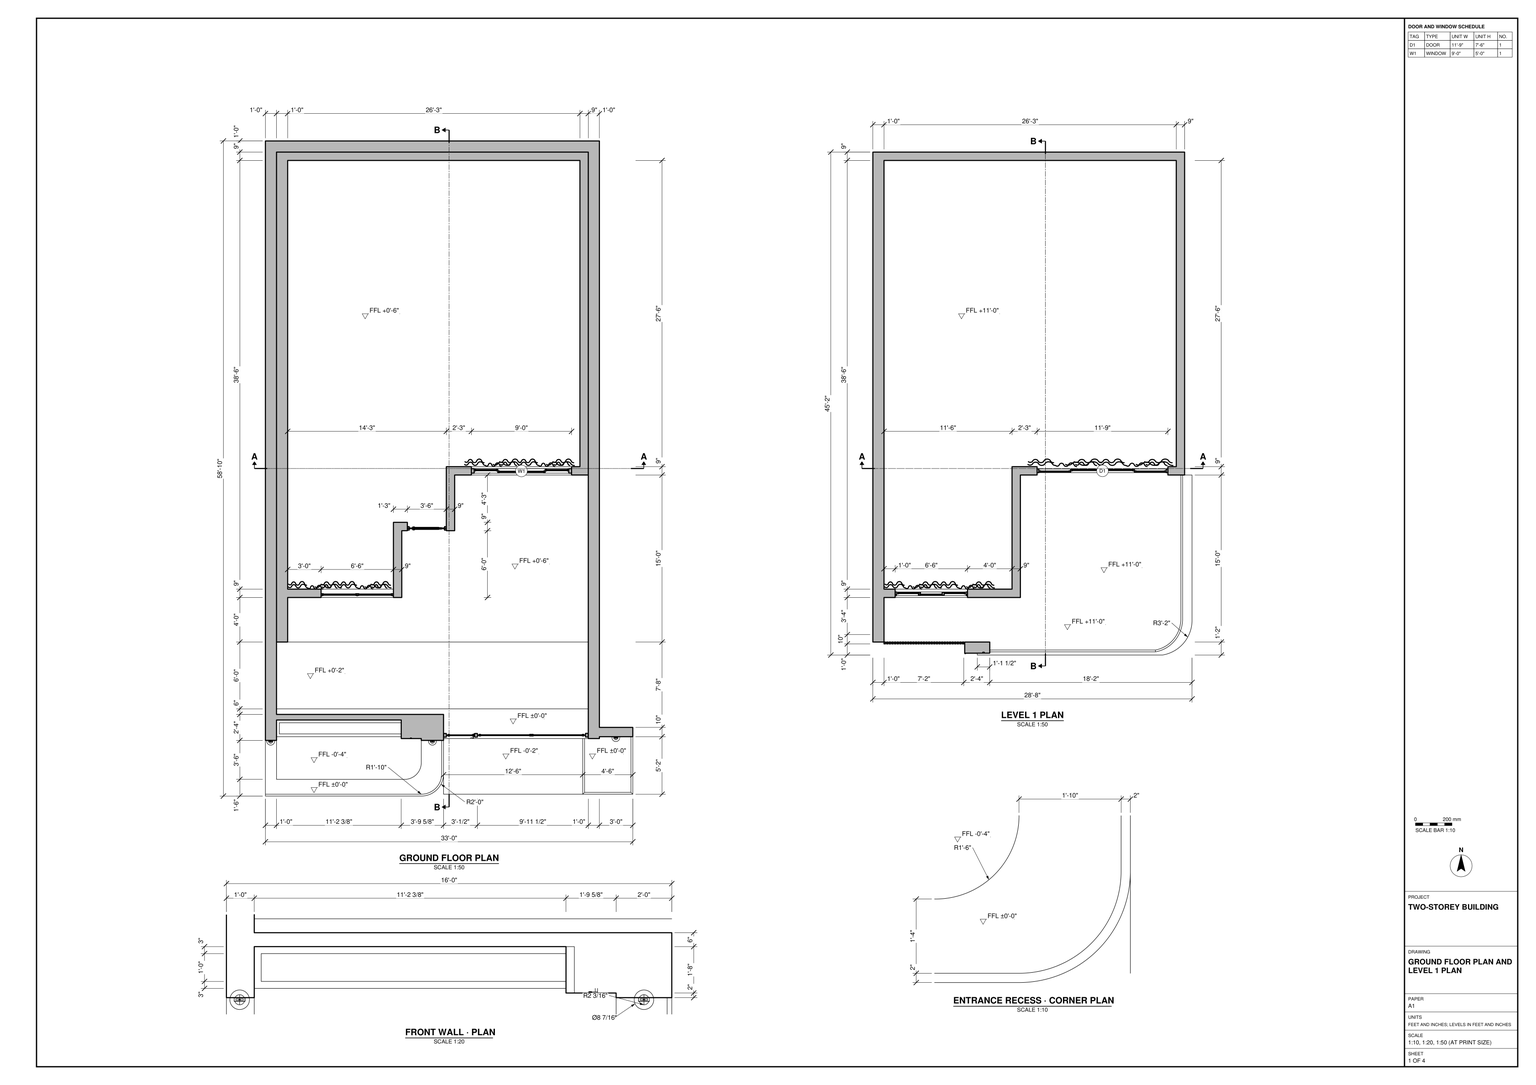
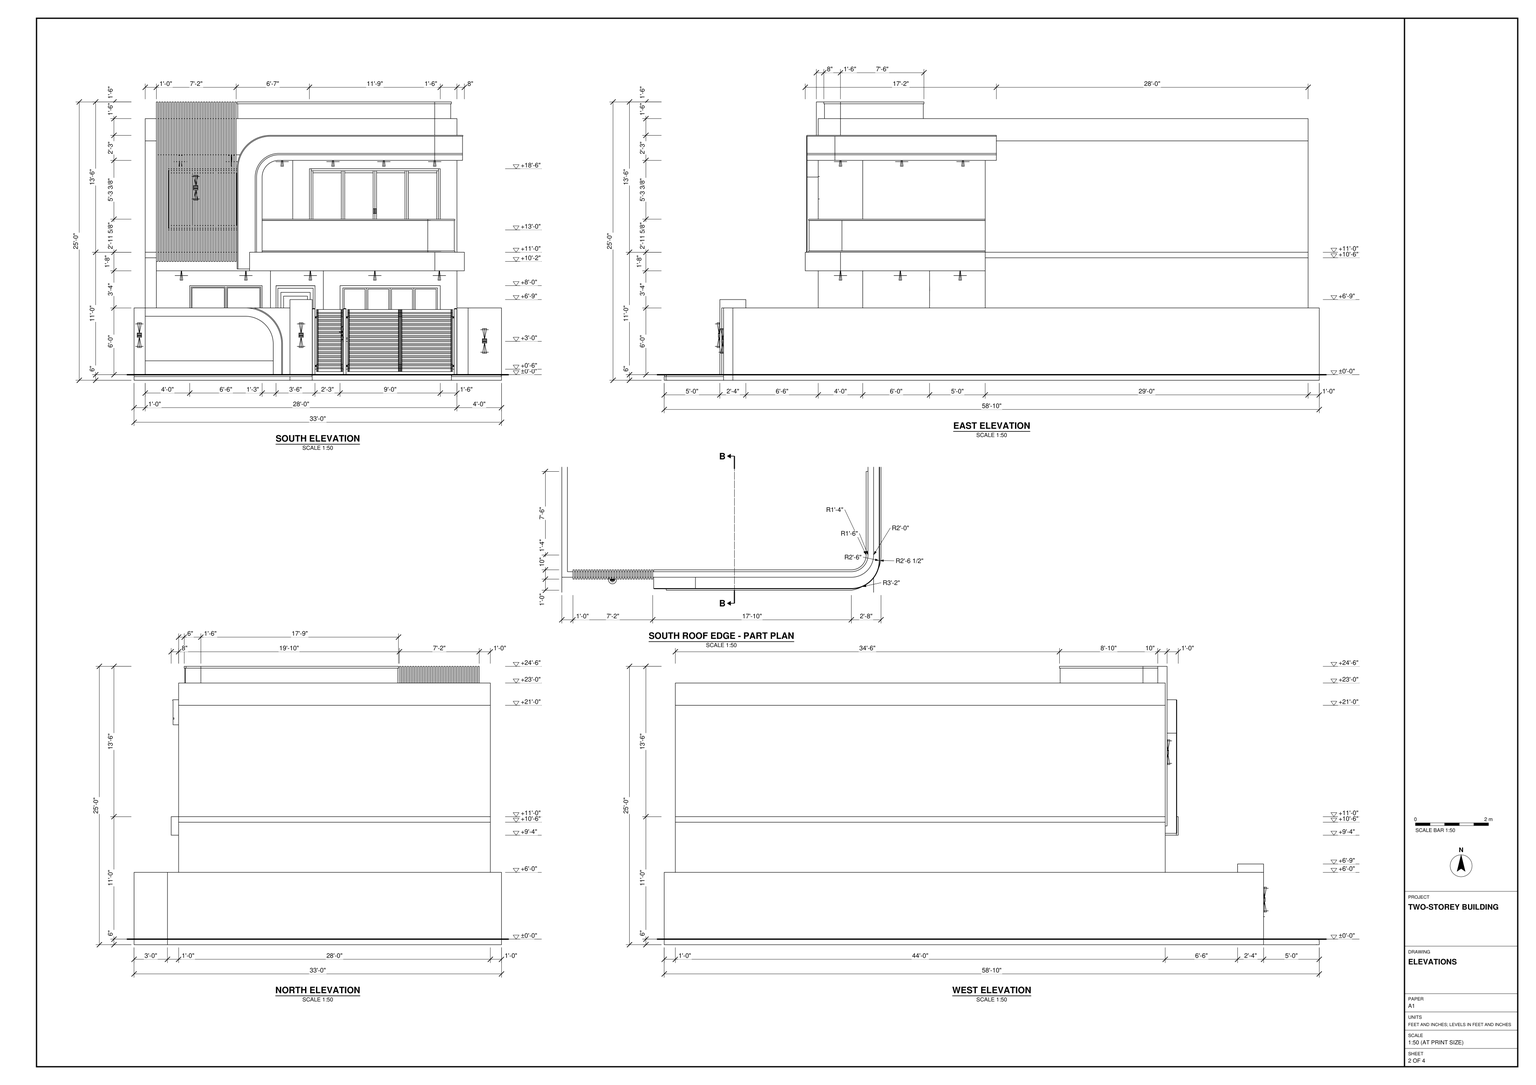
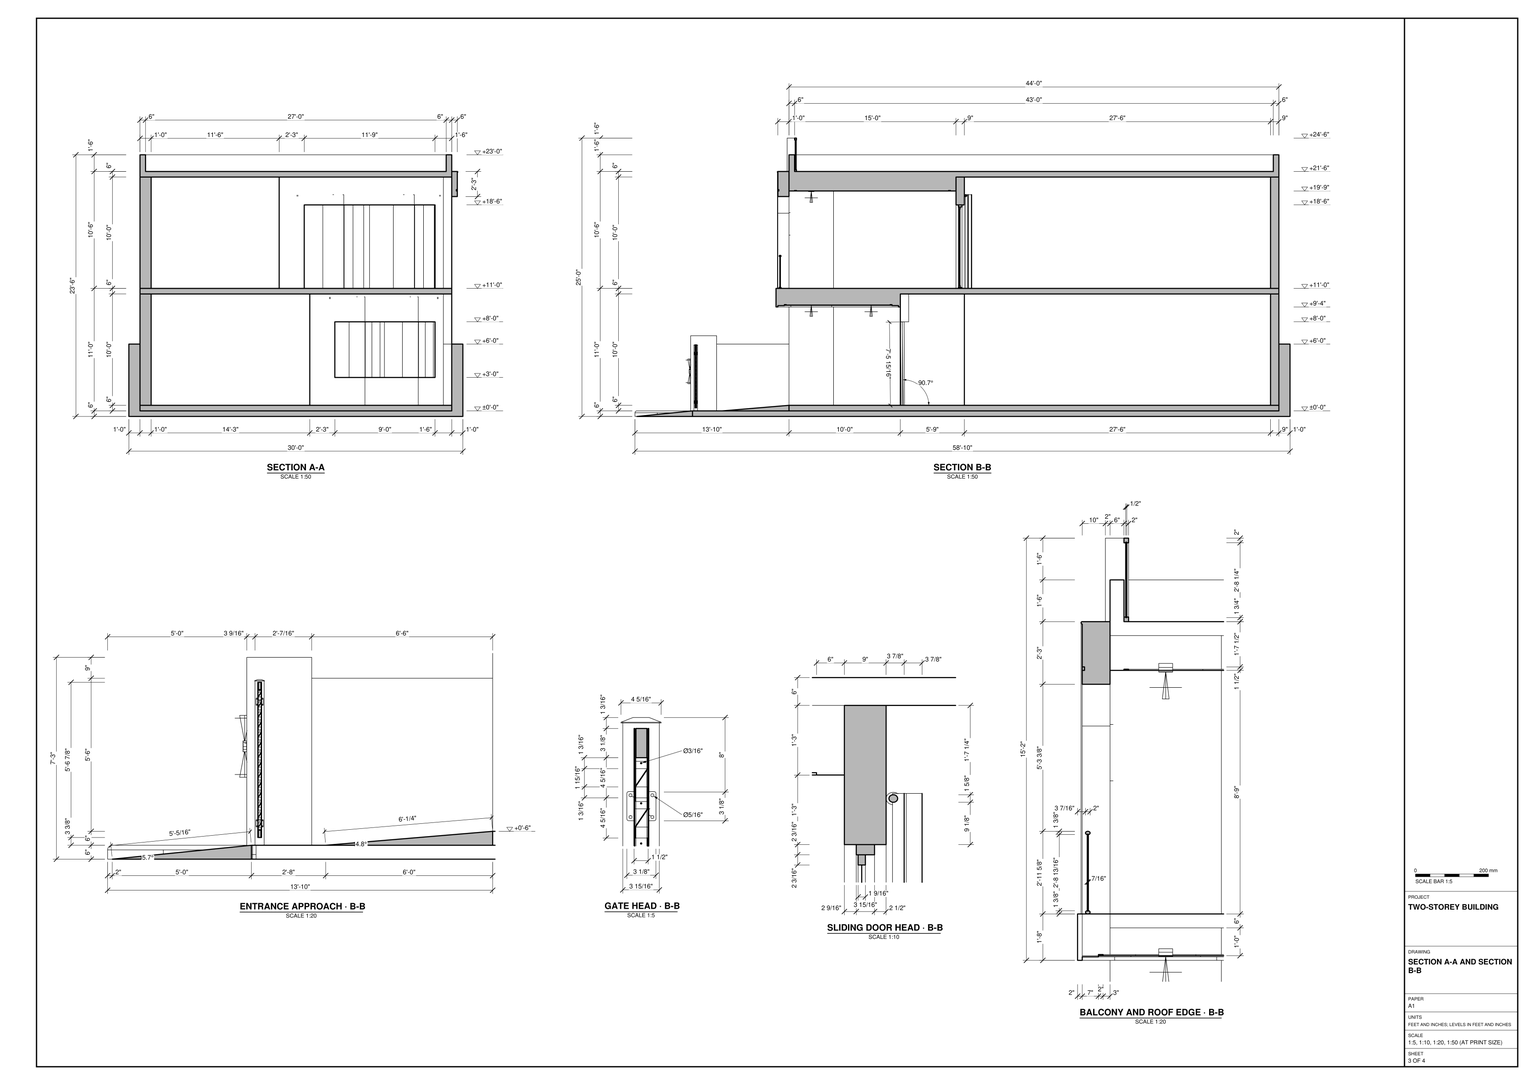
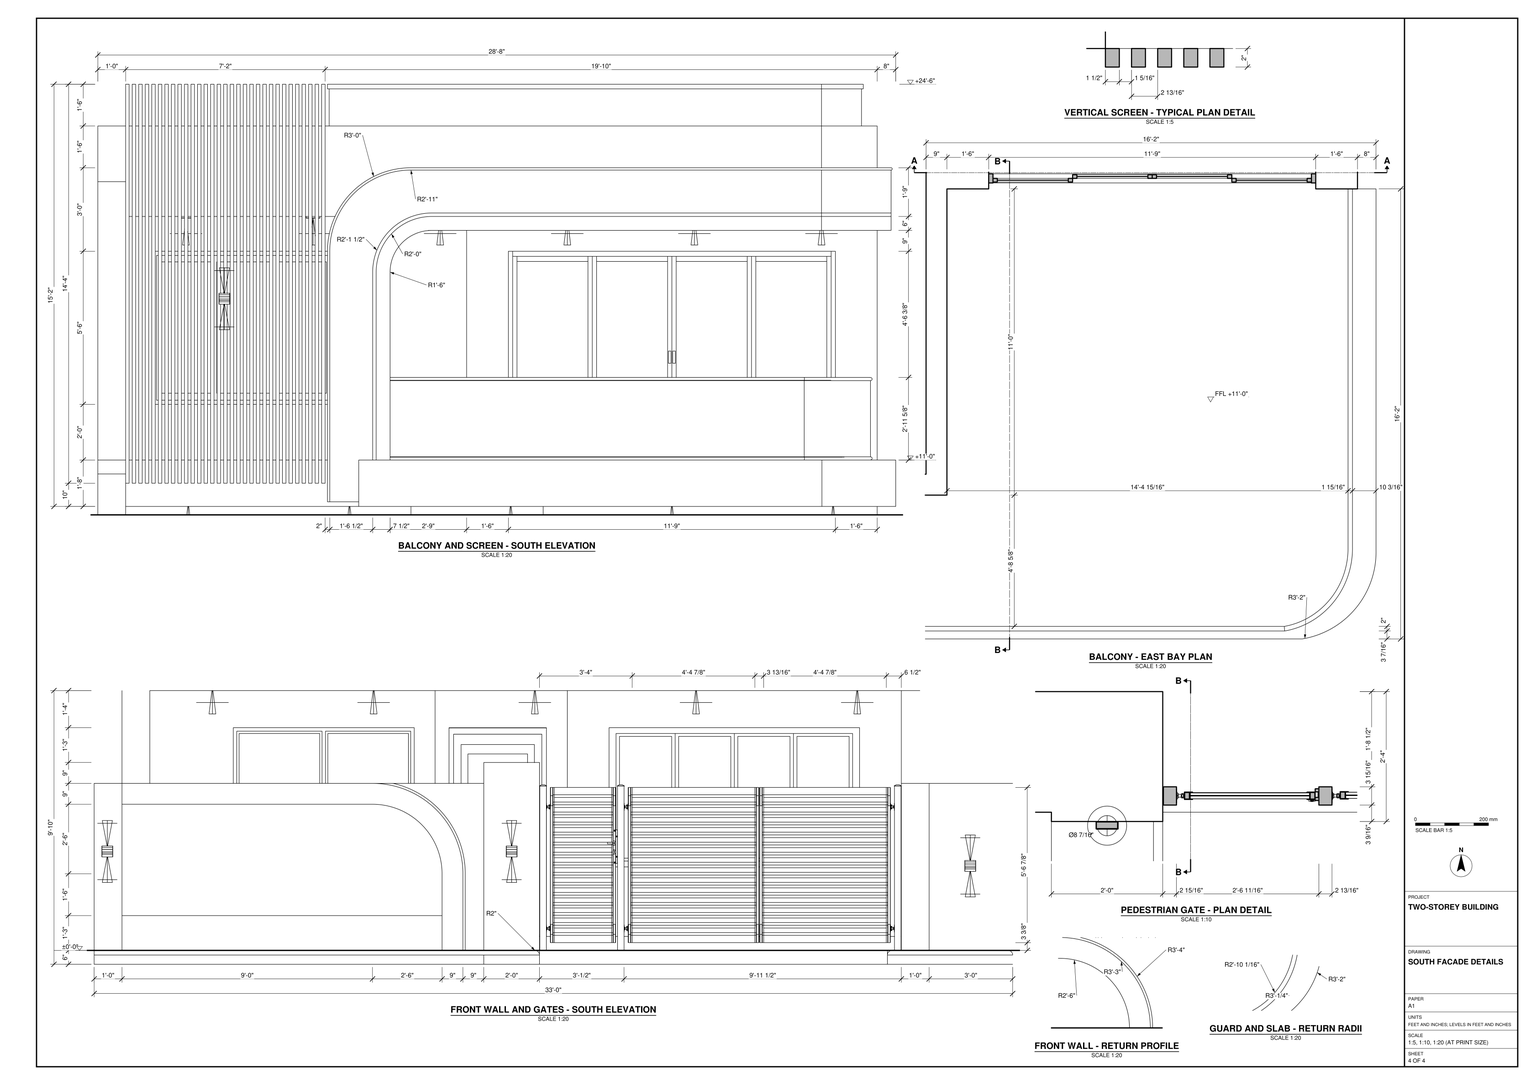
Build the two-storey building and its entrance approach in SketchUp from task_files/diagram_01.pdf. Work in feet and inches. Set the overall width across the south frontage to 33'-0", the front-to-back depth to 58'-10", and the overall height to 25'-0". Use ±0'-0" as the ground-floor datum and +11'-0" as the upper-floor level. Follow the local floor and approach elevations shown in plan and section.

Lay out the exterior walls at their drawn thicknesses, distinguishing the 1'-0" west wall from the 9" east wall. Follow the stepped south wall on each floor: the ground-floor entrance and windows sit behind the front gate, and the upper sliding door opens onto the balcony. Model the floor slabs, projecting balcony with its guard and rounded outer corner, and flat roof with its parapet. Use the south elevation to place the vertical screen on the left and shape the curved frame that rises beside it and continues over the balcony. Include the low perimeter walls, recessed front wall, slatted gate and sloping approach in their plan positions.

Keep walls, slabs, roof, and any furniture or joinery pieces in separate groups or components; use components for repeated parts. Decor and loose items, including lights, may be any suitable library components placed as shown. Save one SketchUp model as output_files/two_storey_building_with_a_curved_front_balcony.skp.

# SketchUp Ruby script. Lengths in inches.
U = 1.inch
M = Sketchup.active_model
def pt(a) = Geom::Point3d.new(a.map { |v| v * U })
def face(e, loops, mat)
  f = e.add_face(loops[0].map { |a| pt(a) })
  loops[1..].each { |l| e.add_face(l.map { |a| pt(a) }).erase! }
  f.material = f.back_material = mat if mat
  f
end
# faces: each face lists its corners as indices into pts; further lists are holes
def faces(e, pts, list, mat = nil) = list.each { |f| face(e, (f[0].is_a?(Array) ? f : [f]).map { |l| l.map { |i| pts[i] } }, mat) }
# xy, xz, yz: faces in a plane at the given z, y or x. An outline is a flat list of corners, or four numbers for a rectangle; further outlines are holes
def ring(l) = l.size == 4 ? [[l[0], l[1]], [l[2], l[1]], [l[2], l[3]], [l[0], l[3]]] : l.each_slice(2).to_a
def flat(e, list, mat, &to3) = list.each { |f| face(e, (f[0].is_a?(Array) ? f : [f]).map { |l| ring(l).map { |u, v| to3.(u, v) } }, mat) }
def xy(e, z, list, mat = nil) = flat(e, list, mat) { |x, y| [x, y, z] }
def xz(e, y, list, mat = nil) = flat(e, list, mat) { |x, z| [x, y, z] }
def yz(e, x, list, mat = nil) = flat(e, list, mat) { |y, z| [x, y, z] }
def lines(e, pts, list) = list.each { |a, b| e.add_line(pt(pts[a]), pt(pts[b])) }
# prism: a flat outline (further loops are holes) pulled along v
def prism(e, loops, v, mat = nil)
  f = face(e, loops, mat); d = Geom::Vector3d.new(v.map { |x| x * U })
  f.pushpull(f.normal.samedirection?(d) ? d.length : -d.length)
end
def box(e, o, s, mat = nil) = prism(e, [[o, [o[0] + s[0], o[1], o[2]], [o[0] + s[0], o[1] + s[1], o[2]], [o[0], o[1] + s[1], o[2]]]], [0, 0, s[2]], mat)
def at(x, y, z, deg = 0) = Geom::Transformation.translation(pt([x, y, z])) * Geom::Transformation.rotation(ORIGIN, Z_AXIS, deg.degrees)
def axes(o, x, y, z) = Geom::Transformation.new([*x, 0, *y, 0, *z, 0, *pt(o).to_a, 1])
def part(name) = M.definitions.add(name)
# library, detail: a bought-in or finely detailed component or shape, given as its bounding box
def library(name, o, s) = part(name).tap { |d| box(d.entities, o, s) }
def detail(e, o, s) = box(e.add_group.entities, o, s)
def put(e, d, t, mat = nil) = e.add_instance(d, t).tap { |i| i.material = mat if mat }
def group(e, t, mat = nil) = e.add_group.tap { |g| g.transformation = t; g.material = mat if mat }.entities
root = M.entities
M.materials.add("1432 AP 8245 TAR ROAD").color = [57, 57, 60]
M.materials.add("Carpet_Frieze_Low").color = [170, 156, 146]
M.materials.add("Carpet_Loop_Low").color = [201, 172, 127]
M.materials.add("[Brick_Pavers_Herringbone]").color = [34, 34, 36]
M.materials.add("[Marble Carrara Floor Tile]").color = [204, 208, 219]
M.materials.add("[Metal_Corrogated_Shiny]").color = [193, 193, 193]
M.materials.add("[Metal_Steel_Textured]").color = [106, 110, 123]
M.materials.add("[Steel Brushed Stainless]").color = [71, 71, 71]
M.materials.add("[Translucent Glass Blue]").color = [188, 212, 255]
M.materials.add("[Translucent Glass Gray]").color = [128, 128, 128]
M.materials.add("[Translucent_Glass_Gray]").color = [128, 128, 128]
M.materials.add("[Wood Veneer 01]").color = [99, 65, 42]
M.materials.add("[Wood_Board_Cork]1").color = [15, 14, 15]
c1 = library("WALL LIGHT 61",[-1.86,-2.6875,-10.98],[8.43,8.43,26.69])
c2 = library("Group\#15",[-12,-57,-27.32],[336,528,69.32])
c3 = library("Group\#14",[-12,-71,-24.08],[344,542,156.08])
c4 = part("Group\#13")
box(c4.entities,[0,0,0],[1.97,3.9375,10.02])
c5 = part("Group\#9")
box(c5.entities,[0,2.36,0.1],[1.97,1.58,9.67])
c6 = part("Group\#10")
xz(c6.entities,0,[[0,0,33.34,51.88]])
c7 = part("Group\#11")
xy(c7.entities,0.1,[[0,2.36,1.97,3.9375]])
xy(c7.entities,4.64,[[0.39,2.36,1.57,2.95]])
xy(c7.entities,5.23,[[0.39,2.36,1.57,2.95]])
xy(c7.entities,9.77,[[0,2.36,1.97,3.9375]])
xz(c7.entities,2.36,[[[0,0.1,1.97,9.77],[0.39,4.64,1.57,5.23]]])
xz(c7.entities,2.95,[[0.39,4.64,1.57,5.23]])
xz(c7.entities,3.9375,[[0,0.1,1.97,9.77]])
yz(c7.entities,0,[[2.36,0.1,3.9375,9.77]])
yz(c7.entities,0.39,[[2.36,4.64,2.95,5.23]])
yz(c7.entities,1.57,[[2.36,4.64,2.95,5.23]])
yz(c7.entities,1.97,[[2.36,0.1,3.9375,9.77]])
c8 = part("slide door")
p = [[0,0,0],[118.11,0,0],[0,0,80.71],[0,-3.9375,80.71],[93.24,-3.9375,80.71]]
lines(c8.entities,p,[[0,1],[2,0],[3,4]])
put(c8.entities,c4,axes([116.56,-3.9375,0],[0.78947,0,0],[0,1,0],[0,0,8.05818]))
put(c8.entities,c4,axes([0,-3.9375,0],[0.78947,0,0],[0,1,0],[0,0,8.05818]))
put(c8.entities,c4,axes([1.55,-3.9375,80.71],[0,0,-1],[0,1,0],[11.48213,0,0]))
g1 = group(c8.entities,at(1.55,-3.9375,1.97))
box(g1,[0,0,-1.97],[115,3.9375,0.79])
put(c8.entities,c5,axes([1.55,-5.91,0],[0.78947,0,0],[0,1,0],[0,0,8.05818]))
put(c8.entities,c5,axes([28.75,-5.91,0],[0.78947,0,0],[0,1,0],[0,0,8.05818]))
put(c8.entities,c5,axes([2.85,-5.91,2.76],[0,0,-1],[0,1,0],[2.65072,0,0]))
put(c8.entities,c5,axes([2.85,-5.91,78.74],[0,0,-1],[0,1,0],[2.65072,0,0]))
put(c8.entities,c6,axes([3.11,-2.76,2.76],[0.76906,0,0],[0,1,0],[0,0,1.42673]),"[Translucent Glass Gray]")
put(c8.entities,c5,axes([89.1,-5.91,78.74],[0,0,-1],[0,1,0],[2.65072,0,0]))
put(c8.entities,c6,axes([89.36,-2.76,2.76],[0.76906,0,0],[0,1,0],[0,0,1.42673]),"[Translucent Glass Gray]")
put(c8.entities,c5,axes([89.1,-5.91,2.76],[0,0,-1],[0,1,0],[2.65072,0,0]))
put(c8.entities,c5,axes([115,-5.91,0],[0.78947,0,0],[0,1,0],[0,0,8.05818]))
put(c8.entities,c5,axes([87.81,-5.91,0],[0.78947,0,0],[0,1,0],[0,0,8.05818]))
put(c8.entities,c6,axes([31.86,-1.18,2.76],[0.76906,0,0],[0,1,0],[0,0,1.42673]),"[Translucent Glass Gray]")
put(c8.entities,c5,axes([31.6,-4.33,78.74],[0,0,-1],[0,1,0],[2.65072,0,0]))
put(c8.entities,c7,axes([57.5,-4.33,0],[0.78947,0,0],[0,1,0],[0,0,8.05818]))
put(c8.entities,c5,axes([31.6,-4.33,2.76],[0,0,-1],[0,1,0],[2.65072,0,0]))
put(c8.entities,c5,axes([30.3,-4.33,0],[0.78947,0,0],[0,1,0],[0,0,8.05818]))
put(c8.entities,c5,axes([87.81,-4.33,0],[-0.78947,0,0],[0,1,0],[0,0,8.05818]))
put(c8.entities,c7,axes([60.61,-4.33,0],[-0.78947,0,0],[0,1,0],[0,0,8.05818]))
put(c8.entities,c5,axes([86.51,-4.33,2.76],[0,0,-1],[0,1,0],[-2.65072,0,0]))
put(c8.entities,c5,axes([86.51,-4.33,78.74],[0,0,-1],[0,1,0],[-2.65072,0,0]))
put(c8.entities,c6,axes([86.25,-1.18,2.76],[-0.76906,0,0],[0,1,0],[0,0,1.42673]),"[Translucent Glass Gray]")
c9 = part("Curtain panel")
# 43 loose lines left out
p = [[17.625,0.0625,78.74],[17.625,0.0625,0],[18.27,0,0],[18.27,0,78.74],[18.92,0.0625,0],[18.92,0.0625,78.74],
  [17,0.25,78.74],[17,0.25,0],[19.55,0.25,0],[19.55,0.25,78.74],[16.43,0.56,78.74],[16.43,0.56,0],
  [20.12,0.56,0],[20.12,0.56,78.74],[6.31,0.6,78.74],[6.31,0.6,0],[6.8125,0.45,0],[6.8125,0.45,78.74],
  [7.33,0.4,0],[7.33,0.4,78.74],[7.86,0.45,0],[7.86,0.45,78.74],[8.36,0.6,0],[8.36,0.6,78.74],
  [5.85,0.85,78.74],[5.85,0.85,0],[8.82,0.85,0],[8.82,0.85,78.74],[15.92,0.97,78.74],[15.92,0.97,0],
  [20.625,0.97,0],[20.625,0.97,78.74],[5.44,1.18,78.74],[5.44,1.18,0],[9.23,1.18,0],[9.23,1.18,78.74],
  [15.51,1.48,78.74],[15.51,1.48,0],[21.04,1.48,0],[21.04,1.48,78.74],[5.11,1.59,78.74],[5.11,1.59,0],
  [9.5625,1.59,0],[9.5625,1.59,78.74],[14.93,2.55,78.74],[14.93,2.55,0],[15.2,2.04,0],[15.2,2.04,78.74],
  [21.34,2.04,0],[21.64,2.59,0],[21.64,2.59,78.74],[21.34,2.04,78.74],[4.63,2.47,78.74],[4.63,2.47,0],
  [4.86,2.04,0],[4.86,2.04,78.74],[9.81,2.04,0],[10.08,2.55,0],[10.08,2.55,78.74],[9.81,2.04,78.74],
  [4.32,2.85,78.74],[4.32,2.85,0],[10.44,2.99,0],[10.44,2.99,78.74],[14.57,2.99,78.74],[14.57,2.99,0],
  [22.03,3.0625,0],[22.03,3.0625,78.74],[0.85,2.85,78.74],[0.85,2.85,0],[1.22,3.15,0],[1.22,3.15,78.74],
  [3.95,3.15,78.74],[3.95,3.15,0],[10.89,3.35,0],[10.89,3.35,78.74],[14.125,3.35,78.74],[14.125,3.35,0],
  [22.5,3.45,0],[22.5,3.45,78.74],[1.65,3.375,0],[1.65,3.375,78.74],[3.53,3.375,78.74],[3.53,3.375,0],
  [2.11,3.52,0],[2.11,3.52,78.74],[3.07,3.52,78.74],[3.07,3.52,0],[11.39,3.625,0],[11.39,3.625,78.74],
  [13.62,3.625,78.74],[13.62,3.625,0],[2.59,3.5625,0],[2.59,3.5625,78.74],[23.04,3.74,0],[23.04,3.74,78.74],
  [11.9375,3.79,0],[11.9375,3.79,78.74],[13.07,3.79,78.74],[13.07,3.79,0],[23.63,3.92,0],[23.63,3.92,78.74],
  [12.51,3.85,0],[12.51,3.85,78.74],[24.25,3.98,0],[24.25,3.98,78.74]]
faces(c9.entities,p,[[0,1,2,3],[3,2,4,5],[6,7,1,0],[5,4,8,9],[10,11,7,6],[9,8,12,13],[14,15,16,17],[17,16,18,19],
  [19,18,20,21],[21,20,22,23],[24,25,15,14],[23,22,26,27],[28,29,11,10],[13,12,30,31],[32,33,25,24],[27,26,34,35],
  [36,37,29,28],[31,30,38,39],[40,41,33,32],[35,34,42,43],[44,45,46,37,36,47],[39,38,48,49,50,51],[52,53,54,41,40,55],[43,42,56,57,58,59],
  [60,61,53,52],[58,57,62,63],[64,65,45,44],[50,49,66,67],[68,69,70,71],[72,73,61,60],[63,62,74,75],[76,77,65,64],
  [67,66,78,79],[71,70,80,81],[82,83,73,72],[81,80,84,85],[86,87,83,82],[75,74,88,89],[90,91,77,76],[85,84,92,93],
  [93,92,87,86],[79,78,94,95],[89,88,96,97],[98,99,91,90],[95,94,100,101],[97,96,102,103],[103,102,99,98],[101,100,104,105]])
c10 = part("Curtain rod section")
yz(c10.entities,0,[[1.55,0.61,1.31,0.64,1.08,0.73,0.88,0.88,0.73,1.08,0.64,1.31,0.61,1.55,0.64,1.79,0.73,2.02,0.88,2.22,1.08,2.37,1.31,2.46,1.55,2.49,1.79,2.46,2.02,2.37,2.22,2.22,2.37,2.02,2.46,1.79,2.49,1.55,2.46,1.31,2.37,1.08,2.22,0.88,2.02,0.73,1.79,0.64]])
yz(c10.entities,2.36,[[[1.55,0,1.15,0.05,0.78,0.21,0.45,0.45,0.21,0.78,0.05,1.15,0,1.55,0.05,1.95,0.21,2.33,0.45,2.65,0.78,2.89,1.15,3.05,1.55,3.1,1.95,3.05,2.33,2.89,2.65,2.65,2.89,2.33,3.05,1.95,3.1,1.55,3.05,1.15,2.89,0.78,2.65,0.45,2.33,0.21,1.95,0.05],[1.55,0.61,1.79,0.64,2.02,0.73,2.22,0.88,2.37,1.08,2.46,1.31,2.49,1.55,2.46,1.79,2.37,2.02,2.22,2.22,2.02,2.37,1.79,2.46,1.55,2.49,1.31,2.46,1.08,2.37,0.88,2.22,0.73,2.02,0.64,1.79,0.61,1.55,0.64,1.31,0.73,1.08,0.88,0.88,1.08,0.73,1.31,0.64]]])
yz(c10.entities,3.15,[[[1.55,0,1.95,0.05,2.33,0.21,2.65,0.45,2.89,0.78,3.05,1.15,3.1,1.55,3.05,1.95,2.89,2.33,2.65,2.65,2.33,2.89,1.95,3.05,1.55,3.1,1.15,3.05,0.78,2.89,0.45,2.65,0.21,2.33,0.05,1.95,0,1.55,0.05,1.15,0.21,0.78,0.45,0.45,0.78,0.21,1.15,0.05],[1.55,0.61,1.31,0.64,1.08,0.73,0.88,0.88,0.73,1.08,0.64,1.31,0.61,1.55,0.64,1.79,0.73,2.02,0.88,2.22,1.08,2.37,1.31,2.46,1.55,2.49,1.79,2.46,2.02,2.37,2.22,2.22,2.37,2.02,2.46,1.79,2.49,1.55,2.46,1.31,2.37,1.08,2.22,0.88,2.02,0.73,1.79,0.64]]])
yz(c10.entities,61.24,[[1.55,0.61,1.79,0.64,2.02,0.73,2.22,0.88,2.37,1.08,2.46,1.31,2.49,1.55,2.46,1.79,2.37,2.02,2.22,2.22,2.02,2.37,1.79,2.46,1.55,2.49,1.31,2.46,1.08,2.37,0.88,2.22,0.73,2.02,0.64,1.79,0.61,1.55,0.64,1.31,0.73,1.08,0.88,0.88,1.08,0.73,1.31,0.64]])
p = [[2.36,1.15,0.05],[2.36,1.55,0],[3.15,1.55,0],[3.15,1.15,0.05],[2.36,1.95,0.05],[3.15,1.95,0.05],
  [2.36,0.78,0.21],[3.15,0.78,0.21],[2.36,2.33,0.21],[3.15,2.33,0.21],[2.36,0.45,0.45],[3.15,0.45,0.45],
  [2.36,2.65,0.45],[3.15,2.65,0.45],[2.36,0.21,0.78],[3.15,0.21,0.78],[2.36,2.89,0.78],[3.15,2.89,0.78],
  [2.36,1.31,0.64],[2.36,1.08,0.73],[0,1.08,0.73],[0,1.31,0.64],[3.15,1.31,0.64],[3.15,1.08,0.73],
  [61.24,1.31,0.64],[61.24,1.08,0.73],[2.36,1.55,0.61],[0,1.55,0.61],[3.15,1.55,0.61],[61.24,1.55,0.61],
  [2.36,1.79,0.64],[0,1.79,0.64],[3.15,1.79,0.64],[61.24,1.79,0.64],[2.36,2.02,0.73],[0,2.02,0.73],
  [3.15,2.02,0.73],[61.24,2.02,0.73],[2.36,0.88,0.88],[0,0.88,0.88],[3.15,0.88,0.88],[61.24,0.88,0.88],
  [2.36,2.22,0.88],[0,2.22,0.88],[3.15,2.22,0.88],[61.24,2.22,0.88],[2.36,0.05,1.15],[3.15,0.05,1.15],
  [2.36,3.05,1.15],[3.15,3.05,1.15],[2.36,0.73,1.08],[0,0.73,1.08],[3.15,0.73,1.08],[61.24,0.73,1.08],
  [2.36,2.37,1.08],[0,2.37,1.08],[3.15,2.37,1.08],[61.24,2.37,1.08],[2.36,0,1.55],[3.15,0,1.55],
  [2.36,0.64,1.31],[0,0.64,1.31],[3.15,0.64,1.31],[61.24,0.64,1.31],[2.36,2.46,1.31],[0,2.46,1.31],
  [3.15,2.46,1.31],[61.24,2.46,1.31],[2.36,3.1,1.55],[3.15,3.1,1.55],[2.36,0.61,1.55],[0,0.61,1.55],
  [3.15,0.61,1.55],[61.24,0.61,1.55],[2.36,2.49,1.55],[0,2.49,1.55],[3.15,2.49,1.55],[61.24,2.49,1.55],
  [2.36,0.05,1.95],[3.15,0.05,1.95],[2.36,0.64,1.79],[0,0.64,1.79],[3.15,0.64,1.79],[61.24,0.64,1.79],
  [2.36,2.46,1.79],[0,2.46,1.79],[3.15,2.46,1.79],[61.24,2.46,1.79],[2.36,3.05,1.95],[3.15,3.05,1.95],
  [2.36,0.73,2.02],[0,0.73,2.02],[3.15,0.73,2.02],[61.24,0.73,2.02],[2.36,2.37,2.02],[0,2.37,2.02],
  [3.15,2.37,2.02],[61.24,2.37,2.02],[2.36,0.21,2.33],[3.15,0.21,2.33],[2.36,0.88,2.22],[0,0.88,2.22],
  [3.15,0.88,2.22],[61.24,0.88,2.22],[2.36,2.22,2.22],[0,2.22,2.22],[3.15,2.22,2.22],[61.24,2.22,2.22],
  [2.36,2.89,2.33],[3.15,2.89,2.33],[2.36,1.08,2.37],[0,1.08,2.37],[3.15,1.08,2.37],[61.24,1.08,2.37],
  [2.36,2.02,2.37],[0,2.02,2.37],[3.15,2.02,2.37],[61.24,2.02,2.37],[2.36,0.45,2.65],[3.15,0.45,2.65],
  [2.36,2.65,2.65],[3.15,2.65,2.65],[2.36,1.31,2.46],[0,1.31,2.46],[3.15,1.31,2.46],[61.24,1.31,2.46],
  [2.36,1.79,2.46],[0,1.79,2.46],[3.15,1.79,2.46],[61.24,1.79,2.46],[2.36,1.55,2.49],[0,1.55,2.49],
  [3.15,1.55,2.49],[61.24,1.55,2.49],[2.36,0.78,2.89],[3.15,0.78,2.89],[2.36,2.33,2.89],[3.15,2.33,2.89],
  [2.36,1.15,3.05],[3.15,1.15,3.05],[2.36,1.95,3.05],[3.15,1.95,3.05],[2.36,1.55,3.1],[3.15,1.55,3.1]]
faces(c10.entities,p,[[0,1,2,3],[1,4,5,2],[6,0,3,7],[4,8,9,5],[10,6,7,11],[8,12,13,9],[14,10,11,15],[12,16,17,13],
  [18,19,20,21],[19,18,22,23],[24,25,23,22],[26,18,21,27],[18,26,28,22],[29,24,22,28],[30,26,27,31],[26,30,32,28],
  [33,29,28,32],[34,30,31,35],[30,34,36,32],[37,33,32,36],[19,38,39,20],[38,19,23,40],[25,41,40,23],[42,34,35,43],
  [34,42,44,36],[45,37,36,44],[46,14,15,47],[16,48,49,17],[38,50,51,39],[50,38,40,52],[41,53,52,40],[54,42,43,55],
  [42,54,56,44],[57,45,44,56],[58,46,47,59],[50,60,61,51],[60,50,52,62],[53,63,62,52],[64,54,55,65],[54,64,66,56],
  [67,57,56,66],[48,68,69,49],[60,70,71,61],[70,60,62,72],[63,73,72,62],[74,64,65,75],[64,74,76,66],[77,67,66,76],
  [78,58,59,79],[70,80,81,71],[80,70,72,82],[73,83,82,72],[84,74,75,85],[74,84,86,76],[87,77,76,86],[68,88,89,69],
  [80,90,91,81],[90,80,82,92],[83,93,92,82],[94,84,85,95],[84,94,96,86],[97,87,86,96],[98,78,79,99],[90,100,101,91],
  [100,90,92,102],[93,103,102,92],[104,94,95,105],[94,104,106,96],[107,97,96,106],[88,108,109,89],[100,110,111,101],[110,100,102,112],
  [103,113,112,102],[114,104,105,115],[104,114,116,106],[117,107,106,116],[118,98,99,119],[108,120,121,109],[110,122,123,111],[122,110,112,124],
  [113,125,124,112],[126,114,115,127],[114,126,128,116],[129,117,116,128],[122,130,131,123],[130,122,124,132],[125,133,132,124],[130,126,127,131],
  [126,130,132,128],[133,129,128,132],[134,118,119,135],[120,136,137,121],[138,134,135,139],[136,140,141,137],[142,138,139,143],[140,142,143,141]])
c11 = part("Curtain rod assembly")
put(c11.entities,c10,axes([3.125,-0.76,-71.54],[0,0,1.25313],[0,1.25313,0],[-1.25313,0,0]))
put(c11.entities,c10,axes([3.125,3.125,81],[0,0,-1.25313],[0,-1.25313,0],[-1.25313,0,0]))
c12 = part("Group\#57")
put(c12.entities,c9,axes([-0.76,0,0],[0.8979,0,0],[0,1,0],[0,0,1]),"Carpet_Frieze_Low")
put(c12.entities,c9,axes([37.23,0,0],[0.9782,0,0],[0,1,0],[0,0,1]),"Carpet_Frieze_Low")
c13 = part("curtain2")
p = [[59.99,12.8,78.74],[59.99,12.8,-38.1875],[60.15,12.52,-38.1875],[60.15,12.52,78.74],[66.72,13.7,-38.1875],[66.72,13.7,78.74],
  [73.91,13.97,78.74],[73.91,13.97,-38.1875],[49.31,14.13,-38.1875],[49.31,14.13,78.74],[2.67,12.52,-38.1875],[2.67,12.52,78.74],
  [-8.17,14.13,-38.1875],[-8.17,14.13,78.74],[2.51,12.8,78.74],[2.51,12.8,-38.1875],[16.42,13.97,78.74],[16.42,13.97,-38.1875],
  [9.24,13.7,-38.1875],[9.24,13.7,78.74]]
lines(c13.entities,p,[[0,1],[2,3],[4,5],[6,7],[8,9],[10,11],[12,13],[14,15],[16,17],[18,19]])
put(c13.entities,c9,axes([64.94,10.15,-38.1875],[0.73,0,0],[0,1,0],[0,0,1.485]),"Carpet_Loop_Low")
put(c13.entities,c9,axes([48.6875,11.28,-38.1875],[0.73,0,0],[0,1,0],[0,0,1.485]),"Carpet_Loop_Low")
put(c13.entities,c9,axes([25.83,10.15,-38.1875],[0.96815,0,0],[0,1,0],[0,0,1.485]),"Carpet_Loop_Low")
put(c13.entities,c9,axes([56.28,10.09,-38.1875],[1.28298,0,0],[0,1,0],[0,0,1.485]),"Carpet_Loop_Low")
put(c13.entities,c11,axes([25.47,12.88,78.42],[0,0,-0.798],[0,0.798,0],[0.798,0,0]))
put(c13.entities,c9,axes([7.46,10.15,-38.1875],[0.73,0,0],[0,1,0],[0,0,1.485]),"Carpet_Loop_Low")
put(c13.entities,c9,axes([-1.2,10.09,-38.1875],[1.28298,0,0],[0,1,0],[0,0,1.485]),"Carpet_Loop_Low")
put(c13.entities,c9,axes([-8.79,11.28,-38.1875],[0.73,0,0],[0,1,0],[0,0,1.485]),"Carpet_Loop_Low")
put(c13.entities,c9,axes([-31.65,10.15,-38.1875],[0.96815,0,0],[0,1,0],[0,0,1.485]),"Carpet_Loop_Low")
put(c13.entities,c12,axes([27.05,7.18,-38.1875],[0.98,0,0],[0,1,0],[0,0,1.485]))
put(c13.entities,c12,axes([-30.43,7.18,-38.1875],[0.98,0,0],[0,1,0],[0,0,1.485]))
c14 = part("Curtains")
put(c14.entities,c13,axes([31.62,15.375,38.1875],[1,0,0],[0,-1,0],[0,0,1]))
c15 = part("porta")
xy(c15.entities,5.98,[[10.33,-5.78,50.62,-5.46]],"[Wood_Board_Cork]1")
xy(c15.entities,36.43,[[47.65,-6.28,49.65,-6.19]],"[Metal_Corrogated_Shiny]")
xy(c15.entities,42.81,[[47.65,-6.37,49.65,-6.28]],"[Metal_Corrogated_Shiny]")
xy(c15.entities,74.08,[[14.08,-7.02,46.87,-6.71]],"[Wood_Board_Cork]1")
yz(c15.entities,3.7,[[-6.9,1.31,-8.04,84.45,-6.04,84.48,-4.9,1.34]],"[Brick_Pavers_Herringbone]")
yz(c15.entities,6.22,[[-6.9,1.31,-4.9,1.34,-4.91,1.875,-5.41,1.87,-6.51,81.95,-8.01,81.93]],"[Brick_Pavers_Herringbone]")
yz(c15.entities,10.33,[[-5.78,5.98,-6.76,77.83,-6.45,77.84,-5.46,5.98]],"[Wood_Board_Cork]1")
yz(c15.entities,14.08,[[-6.14,9.72,-7.02,74.08,-6.71,74.08,-5.83,9.73]],"[Wood_Board_Cork]1")
yz(c15.entities,46.87,[[-6.14,9.72,-5.83,9.73,-6.71,74.08,-7.02,74.08]],"[Wood_Board_Cork]1")
yz(c15.entities,47.65,[[-6.1875,36.06,-6.46,36.61,-6.6875,37.1875,-6.87,37.78,-7,38.38,-7.08,38.99,-7.11,39.61,-7.1,40.22,-7.03,40.84,-6.92,41.44,-6.75,42.04,-6.54,42.62,-6.29,43.18,-6.28,42.81,-6.37,42.81,-6.47,42.59,-6.67,42.01,-6.83,41.43,-6.95,40.83,-7.01,40.22,-7.03,39.61,-7,39,-6.91,38.39,-6.78,37.8,-6.61,37.21,-6.38,36.65,-6.28,36.43,-6.19,36.43]],"[Metal_Corrogated_Shiny]")
yz(c15.entities,48.41,[[-6.03,33.67,-6.03,33.7,-5.91,33.71,-5.91,33.67],[-6.03,33.7,-6.03,33.74,-5.91,33.74,-5.91,33.71]],"[Metal_Steel_Textured]")
yz(c15.entities,49.65,[[-6.1875,36.06,-6.19,36.43,-6.28,36.43,-6.38,36.65,-6.61,37.21,-6.78,37.8,-6.91,38.39,-7,39,-7.03,39.61,-7.01,40.22,-6.95,40.83,-6.83,41.43,-6.67,42.01,-6.47,42.59,-6.37,42.81,-6.28,42.81,-6.29,43.18,-6.54,42.62,-6.75,42.04,-6.92,41.44,-7.03,40.84,-7.1,40.22,-7.11,39.61,-7.08,38.99,-7,38.38,-6.87,37.78,-6.6875,37.1875,-6.46,36.61]],"[Metal_Corrogated_Shiny]")
yz(c15.entities,50.62,[[-5.78,5.98,-5.46,5.98,-6.45,77.84,-6.76,77.83]],"[Wood_Board_Cork]1")
yz(c15.entities,54.73,[[-6.9,1.31,-8.01,81.93,-6.51,81.95,-5.41,1.87,-4.91,1.875,-4.9,1.34]],"[Brick_Pavers_Herringbone]")
yz(c15.entities,57.25,[[-6.9,1.31,-4.9,1.34,-6.04,84.48,-8.04,84.45]],"[Brick_Pavers_Herringbone]")
p = [[3.7,-6.9,1.31],[6.22,-6.9,1.31],[6.22,-8.01,81.93],[54.73,-8.01,81.93],[54.73,-6.9,1.31],[57.25,-6.9,1.31],
  [57.25,-8.04,84.45],[3.7,-8.04,84.45],[3.7,-4.9,1.34],[6.22,-4.9,1.34],[54.73,-4.9,1.34],[57.25,-4.9,1.34],
  [3.7,-6.04,84.48],[57.25,-6.04,84.48],[54.73,-4.91,1.875],[6.22,-4.91,1.875],[6.22,-6.51,81.95],[6.22,-5.41,1.87],
  [54.73,-5.41,1.87],[54.73,-6.51,81.95],[50.62,-6.45,77.84],[50.62,-5.46,5.98],[10.33,-5.46,5.98],[10.33,-6.45,77.84],
  [50.62,-5.78,5.98],[50.62,-6.76,77.83],[10.33,-6.76,77.83],[10.33,-5.78,5.98],[46.87,-5.83,9.73],[14.08,-5.83,9.73],
  [14.08,-6.71,74.08],[46.87,-6.71,74.08],[48.72,-6.15,33.45],[48.64,-6.15,33.35],[48.54,-6.15,33.27],[48.42,-6.15,33.22],
  [48.29,-6.15,33.2],[48.16,-6.15,33.22],[48.04,-6.15,33.27],[47.93,-6.15,33.35],[47.85,-6.15,33.45],[47.8,-6.15,33.57],
  [47.79,-6.16,33.7],[47.8,-6.16,33.83],[47.85,-6.16,33.95],[47.93,-6.16,34.06],[48.04,-6.16,34.14],[48.16,-6.16,34.1875],
  [48.29,-6.16,34.2],[48.42,-6.16,34.1875],[48.54,-6.16,34.14],[48.64,-6.16,34.06],[48.72,-6.16,33.95],[48.77,-6.16,33.83],
  [48.79,-6.16,33.7],[48.77,-6.15,33.57],[47.65,-6.1875,36.06],[47.65,-6.19,36.43],[49.65,-6.19,36.43],[49.65,-6.1875,36.06],
  [49.65,-6.28,42.81],[47.65,-6.28,42.81],[47.65,-6.29,43.18],[49.65,-6.29,43.18],[14.08,-6.14,9.72],[46.87,-6.14,9.72],
  [46.87,-7.02,74.08],[14.08,-7.02,74.08],[48.16,-6.03,33.22],[48.04,-6.03,33.27],[48.29,-6.02,33.2],[48.42,-6.03,33.22],
  [48.54,-6.03,33.27],[48.64,-6.03,33.35],[48.72,-6.03,33.45],[48.77,-6.03,33.58],[48.79,-6.03,33.7],[48.77,-6.03,33.83],
  [48.72,-6.04,33.95],[48.64,-6.04,34.06],[48.54,-6.04,34.14],[48.42,-6.04,34.1875],[48.29,-6.04,34.2],[48.16,-6.04,34.1875],
  [48.04,-6.04,34.14],[47.93,-6.04,34.06],[47.85,-6.04,33.95],[47.8,-6.03,33.83],[47.79,-6.03,33.7],[47.8,-6.03,33.58],
  [47.85,-6.03,33.45],[47.93,-6.03,33.35],[48.39,-6.03,33.77],[48.41,-6.03,33.74],[48.41,-6.03,33.7],[48.41,-6.03,33.67],
  [48.39,-6.03,33.64],[48.375,-6.03,33.62],[48.35,-6.03,33.6],[48.32,-6.03,33.59],[48.29,-6.03,33.58],[48.26,-6.03,33.59],
  [48.23,-6.03,33.6],[48.2,-6.03,33.62],[48.18,-6.03,33.64],[48.17,-6.03,33.67],[48.16,-6.03,33.7],[48.17,-6.03,33.74],
  [48.18,-6.03,33.77],[48.2,-6.03,33.79],[48.23,-6.03,33.8125],[48.26,-6.03,33.82],[48.29,-6.03,33.83],[48.32,-6.03,33.82],
  [48.35,-6.03,33.8125],[48.375,-6.03,33.79],[48.18,-5.91,33.65],[48.17,-5.91,33.67],[48.2,-5.91,33.62],[48.23,-5.91,33.6],
  [48.26,-5.91,33.59],[48.29,-5.9,33.58],[48.32,-5.91,33.59],[48.35,-5.91,33.6],[48.375,-5.91,33.62],[48.39,-5.91,33.65],
  [48.41,-5.91,33.67],[48.41,-5.91,33.74],[48.39,-5.91,33.77],[48.375,-5.91,33.79],[48.35,-5.91,33.8125],[48.32,-5.91,33.82],
  [48.29,-5.91,33.83],[48.26,-5.91,33.82],[48.23,-5.91,33.8125],[48.2,-5.91,33.79],[48.18,-5.91,33.77],[48.17,-5.91,33.74],
  [48.16,-5.91,33.71],[48.41,-5.91,33.71],[47.65,-6.46,36.61],[49.65,-6.46,36.61],[47.65,-6.28,36.43],[47.65,-6.38,36.65],
  [49.65,-6.38,36.65],[49.65,-6.28,36.43],[47.65,-6.6875,37.1875],[49.65,-6.6875,37.1875],[47.65,-6.61,37.21],[49.65,-6.61,37.21],
  [47.65,-6.87,37.78],[49.65,-6.87,37.78],[47.65,-6.78,37.8],[49.65,-6.78,37.8],[47.65,-7,38.38],[49.65,-7,38.38],
  [47.65,-6.91,38.39],[49.65,-6.91,38.39],[47.65,-7.08,38.99],[49.65,-7.08,38.99],[47.65,-7,39],[49.65,-7,39],
  [47.65,-7.11,39.61],[49.65,-7.11,39.61],[47.65,-7.03,39.61],[49.65,-7.03,39.61],[47.65,-7.1,40.22],[49.65,-7.1,40.22],
  [47.65,-7.01,40.22],[49.65,-7.01,40.22],[47.65,-7.03,40.84],[49.65,-7.03,40.84],[47.65,-6.95,40.83],[49.65,-6.95,40.83],
  [47.65,-6.92,41.44],[49.65,-6.92,41.44],[47.65,-6.83,41.43],[49.65,-6.83,41.43],[47.65,-6.75,42.04],[49.65,-6.75,42.04],
  [47.65,-6.67,42.01],[49.65,-6.67,42.01],[47.65,-6.54,42.62],[49.65,-6.54,42.62],[47.65,-6.47,42.59],[49.65,-6.47,42.59],
  [47.65,-6.37,42.81],[49.65,-6.37,42.81]]
faces(c15.entities,p,[[0,1,2,3,4,5,6,7],[65,64,29,28],[20,23,26,25]],"[Wood_Board_Cork]1")
faces(c15.entities,p,[[8,9,1,0],[4,10,11,5],[12,13,11,10,14,15,9,8],[[16,17,18,19],[20,21,22,23]],[18,17,15,14],[[24,25,26,27],[28,29,30,31],[32,33,34,35,36,37,38,39,40,41,42,43,44,45,46,47,48,49,50,51,52,53,54,55],[56,57,58,59],[60,61,62,63]],[64,65,66,67],[16,19,3,2],
  [13,12,7,6]],"[Brick_Pavers_Herringbone]")
faces(c15.entities,p,[[38,37,68,69],[37,36,70,68],[36,35,71,70],[35,34,72,71],[[73,74,75,76,77,78,79,80,81,82,83,84,85,86,87,88,89,90,91,69,68,70,71,72],[92,93,94,95,96,97,98,99,100,101,102,103,104,105,106,107,108,109,110,111,112,113,114,115]],[40,39,91,90],[39,38,69,91],[34,33,73,72],
  [33,32,74,73],[41,40,90,89],[32,55,75,74],[42,41,89,88],[55,54,76,75],[43,42,88,87],[54,53,77,76],[44,43,87,86],
  [53,52,78,77],[45,44,86,85],[52,51,79,78],[46,45,85,84],[47,46,84,83],[50,49,81,80],[51,50,80,79],[48,47,83,82],
  [49,48,82,81],[140,56,59,141],[142,143,144,145],[146,140,141,147],[143,148,149,144],[150,146,147,151],[148,152,153,149],[154,150,151,155],
  [152,156,157,153],[158,154,155,159],[156,160,161,157],[162,158,159,163],[160,164,165,161],[166,162,163,167],[164,168,169,165],[170,166,167,171],
  [168,172,173,169],[174,170,171,175],[172,176,177,173],[178,174,175,179],[176,180,181,177],[182,178,179,183],[180,184,185,181],[62,182,183,63],
  [184,186,187,185]],"[Metal_Corrogated_Shiny]")
faces(c15.entities,p,[[105,104,116,117],[104,103,118,116],[103,102,119,118],[102,101,120,119],[101,100,121,120],[100,99,122,121],[99,98,123,122],[98,97,124,123],
  [97,96,125,124],[96,95,126,125],[127,128,129,130,131,132,133,134,135,136,137,138,117,116,118,119,120,121,122,123,124,125,126,139],[108,107,137,136],[107,106,138,137],[106,105,117,138],[93,92,128,127],[111,110,134,133],
  [110,109,135,134],[109,108,136,135],[115,114,130,129],[114,113,131,130],[113,112,132,131],[112,111,133,132],[92,115,129,128]],"[Metal_Steel_Textured]")
c16 = part("Component")
put(c16.entities,c15,axes([57.25,4.9,-1.34],[-1,0,0],[0,1,0],[0,0,1]))
put(c16.entities,c15,axes([57.25,-5.48,-1.41],[-1,0,0],[0,-0.99982,-0.0192],[0,-0.0192,0.99982]))
c17 = part("Window frame")
prism(c17.entities,[[[0,70.87,0],[0,0,0],[0,0,47.24],[0,70.87,47.24]],[[0,1.97,1.97],[0,68.9,1.97],[0,68.9,45.28],[0,1.97,45.28]]],[7.875,0,0])
c18 = part("Window sash")
xy(c18.entities,0,[[0,0,3.9375,16.73]])
xy(c18.entities,0.98,[[0,0.98,1.77,15.75],[1.77,0.98,2.85,15.75],[2.85,0.98,3.9375,15.75]])
xy(c18.entities,42.32,[[0,0.98,1.77,15.75],[1.77,0.98,2.85,15.75],[2.85,0.98,3.9375,15.75]])
xy(c18.entities,43.31,[[0,0,3.9375,16.73]])
xz(c18.entities,0,[[0,0,3.9375,43.31]])
xz(c18.entities,0.98,[[0,0.98,1.77,42.32],[1.77,0.98,2.85,42.32],[2.85,0.98,3.9375,42.32]])
xz(c18.entities,15.75,[[0,0.98,1.77,42.32],[1.77,0.98,2.85,42.32],[2.85,0.98,3.9375,42.32]])
xz(c18.entities,16.73,[[0,0,3.9375,43.31]])
yz(c18.entities,0,[[[0,0,16.73,43.31],[0.98,0.98,15.75,42.32]]])
yz(c18.entities,1.77,[[0.98,0.98,15.75,42.32]],"[Translucent_Glass_Gray]")
yz(c18.entities,2.85,[[0.98,0.98,15.75,42.32]],"[Translucent_Glass_Gray]")
yz(c18.entities,3.9375,[[[0,0,16.73,43.31],[0.98,0.98,15.75,42.32]]])
c19 = part("simple window")
p = [[0,68.9,1.97],[0,35.43,1.97]]
lines(c19.entities,p,[[0,1]])
put(c19.entities,c17,at(0,0,0),"[Steel Brushed Stainless]")
put(c19.entities,c18,axes([1.14,52.17,1.97],[0.71,0,0],[0,1,0],[0,0,1]),"[Steel Brushed Stainless]")
put(c19.entities,c18,axes([1.14,1.97,1.97],[0.71,0,0],[0,1,0],[0,0,1]),"[Steel Brushed Stainless]")
put(c19.entities,c18,axes([3.9375,18.7,1.97],[0.71,0,0],[0,1,0],[0,0,1]),"[Steel Brushed Stainless]")
put(c19.entities,c18,axes([3.9375,35.43,1.97],[0.71,0,0],[0,1,0],[0,0,1]),"[Steel Brushed Stainless]")
c20 = part("1")
prism(c20.entities,[[[36.75,0,63],[36.75,0,0],[0,0,0],[0,0,63]],[[1,0,1],[35.75,0,1],[35.75,0,62],[1,0,62]]],[0,-1.25,0])
g2 = group(c20.entities,at(1,-0.4375,1),"[Translucent Glass Gray]")
box(g2,[0,-0.47,0],[34.75,0.47,61])
c21 = part("2")
prism(c21.entities,[[[0,1.5,0],[0,-0.5,0],[0,-0.5,172],[0,9.5,172],[0,9.5,136],[0,7.5,136],[0,7.5,154],[0,1.5,154]]],[1.5,0,0])
c22 = library("Group\#26",[-12,-166,-6],[396,706,87])
g3 = group(root,at(0,50,0))
g4 = group(g3,at(0,-48,-0.03))
put(g4,c1,at(52.21,-4.41,193.2))
put(g4,c2,at(12,57,246.03))
put(g4,c3,at(12,57,120.03))
g5 = group(g4,at(12,57,126.03))
xy(g5,0,[[-12,-57,-12,471,324,471,324,123,306,123,306,132,315,132,315,462,0,462,0,0,138,0,138,132,165,132,165,123,147,123,147,-9,0,-9,0,-57]])
xy(g5,24,[[12,-9,90,0]])
xy(g5,90,[[12,-9,90,0],[165,123,306,132]])
xy(g5,120,[[[-12,-57,0,-57,0,-9,147,-9,147,123,324,123,324,471,-12,471],[0,0,0,462,315,462,315,132,138,132,138,0]]])
xz(g5,-57,[[-12,0,0,120]],"1432 AP 8245 TAR ROAD")
xz(g5,-9,[[[0,0,147,120],[12,24,90,90]]])
xz(g5,0,[[[0,0,138,120],[12,24,90,90]]])
xz(g5,123,[[147,0,165,0,165,90,306,90,306,0,324,0,324,120,147,120]])
xz(g5,132,[[138,0,138,120,315,120,315,0,306,0,306,90,165,90,165,0]])
xz(g5,462,[[0,0,315,120]])
xz(g5,471,[[-12,0,324,120]])
yz(g5,-12,[[-57,0,471,120]])
yz(g5,0,[[0,0,462,120]])
yz(g5,0,[[-57,0,-9,120]],"1432 AP 8245 TAR ROAD")
yz(g5,12,[[-9,24,0,90]])
yz(g5,90,[[-9,24,0,90]])
yz(g5,138,[[0,0,132,120]])
yz(g5,147,[[-9,0,123,120]])
yz(g5,165,[[123,0,132,90]])
yz(g5,306,[[123,0,132,90]])
yz(g5,315,[[132,0,462,120]])
yz(g5,324,[[123,0,471,120]])
put(g5,c8,axes([165,129.5,0],[1.1938,0,0],[0,1,0],[0,0,1.11512]),"[Steel Brushed Stainless]")
put(g5,c14,axes([154.04,132,0],[1.32227,0,0],[0,1,0],[0,0,0.864]))
put(g5,c14,axes([0,0,0],[1,0,0],[0,1,0],[0,0,0.89]))
g6 = group(g5,at(12,-7,24),"[Steel Brushed Stainless]")
xy(g6,0,[[0,0,78,3.9375]])
xy(g6,1.8,[[1.3,0,76.7,0,76.7,1.97,52.87,1.97,52.87,0.39,25.13,0.39,25.13,1.97,1.3,1.97],[25.13,0.39,27.73,1.97],[50.27,0.39,52.87,1.97],[27.3,1.97,50.7,1.97,50.7,3.54,76.7,3.54,76.7,3.9375,1.3,3.9375,1.3,3.54,27.3,3.54]])
xy(g6,4.8,[[27.3,0.39,50.7,1.18],[27.3,1.18,50.7,1.97],[3.47,1.97,25.13,2.76],[52.87,1.97,74.53,2.76],[3.47,2.76,25.13,3.54],
  [52.87,2.76,74.53,3.54]])
xy(g6,61.43,[[27.3,0.39,50.7,1.18],[27.3,1.18,50.7,1.97],[3.47,1.97,25.13,2.76],[52.87,1.97,74.53,2.76],[3.47,2.76,25.13,3.54],
  [52.87,2.76,74.53,3.54]])
xy(g6,64.2,[[1.3,0,1.3,1.97,25.13,1.97,25.13,0.39,52.87,0.39,52.87,1.97,76.7,1.97,76.7,0],[25.13,0.39,52.87,1.97],[1.3,1.97,27.3,3.54],[27.3,1.97,27.3,3.54,1.3,3.54,1.3,3.9375,76.7,3.9375,76.7,3.54,50.7,3.54,50.7,1.97]])
xy(g6,66,[[0,0,78,3.9375]])
xz(g6,0,[[[0,0,78,66],[1.3,1.8,76.7,64.2]]])
xz(g6,0.39,[[[25.13,1.8,52.87,64.2],[27.3,4.8,50.7,61.43]]])
xz(g6,1.18,[[27.3,4.8,50.7,61.43]],"[Translucent Glass Blue]")
xz(g6,1.97,[[1.3,1.8,25.13,1.8,25.13,4.8,3.47,4.8,3.47,61.43,25.13,61.43,25.13,64.2,1.3,64.2],[25.13,1.8,27.3,64.2],[27.3,1.8,50.7,4.8],[52.87,1.8,76.7,1.8,76.7,64.2,52.87,64.2,52.87,61.43,74.53,61.43,74.53,4.8,52.87,4.8],[27.3,61.43,50.7,64.2]])
xz(g6,2.76,[[3.03,61.2,3.47,62.4]])
xz(g6,2.76,[[3.47,4.8,25.13,61.43],[52.87,4.8,74.53,61.43]],"[Translucent Glass Blue]")
xz(g6,3.54,[[[1.3,1.8,27.3,64.2],[3.47,4.8,25.13,61.43]],[[50.7,1.8,76.7,64.2],[52.87,4.8,74.53,61.43]]])
xz(g6,3.9375,[[[0,0,78,66],[1.3,1.8,76.7,64.2]]])
yz(g6,0,[[0,0,3.9375,66]])
yz(g6,1.3,[[0,1.8,1.97,64.2],[3.54,1.8,3.9375,64.2]])
yz(g6,3.47,[[1.97,4.8,2.76,61.43],[2.76,4.8,3.54,61.43]])
yz(g6,25.13,[[0.39,1.8,1.97,64.2],[1.97,4.8,2.76,61.43],[2.76,4.8,3.54,61.43]])
yz(g6,27.3,[[1.97,1.8,3.54,64.2],[0.39,4.8,1.18,61.43],[1.18,4.8,1.97,61.43]])
yz(g6,50.7,[[1.97,1.8,3.54,64.2],[0.39,4.8,1.18,61.43],[1.18,4.8,1.97,61.43]])
yz(g6,52.87,[[0.39,1.8,1.97,64.2],[1.97,4.8,2.76,61.43],[2.76,4.8,3.54,61.43]])
yz(g6,74.53,[[1.97,4.8,2.76,61.43],[2.76,4.8,3.54,61.43]])
yz(g6,76.7,[[0,1.8,1.97,64.2],[3.54,1.8,3.9375,64.2]])
yz(g6,78,[[0,0,3.9375,66]])
# 1 loose lines left out
g7 = group(g4,at(0,48,0.03))
xy(g7,0,[[0,-48,0,480,336,480,336,132,192,132,192,72,183,72,183,141,327,141,327,471,12,471,12,9,126,9,126,81,141,81,141,72,135,72,135,0,12,0,12,-48]])
xy(g7,24,[[48,0,126,9]])
xy(g7,30,[[210,132,318,141]])
xy(g7,90,[[48,0,126,9],[141,72,183,81],[210,132,318,141]])
xy(g7,120,[[[0,-48,12,-48,12,0,135,0,135,72,192,72,192,132,336,132,336,480,0,480],[12,9,12,471,327,471,327,141,183,141,183,81,126,81,126,9]]])
xz(g7,-48,[[0,0,12,120]],"1432 AP 8245 TAR ROAD")
xz(g7,0,[[[12,0,135,120],[48,24,126,90]]])
xz(g7,9,[[12,0,12,120,126,120,126,90,48,90,48,24,126,24,126,0]])
xz(g7,72,[[135,0,141,0,141,90,183,90,183,0,192,0,192,120,135,120]])
xz(g7,81,[[126,0,126,120,183,120,183,90,141,90,141,0]])
xz(g7,132,[[[192,0,336,120],[210,30,318,90]]])
xz(g7,141,[[[183,0,327,120],[210,30,318,90]]])
xz(g7,471,[[12,0,327,120]])
xz(g7,480,[[0,0,336,120]])
yz(g7,0,[[-48,0,480,120]])
yz(g7,12,[[9,0,471,120]])
yz(g7,12,[[-48,0,0,120]],"1432 AP 8245 TAR ROAD")
yz(g7,48,[[0,24,9,90]])
yz(g7,126,[[9,0,81,120],[0,24,9,90]])
yz(g7,135,[[0,0,72,120]])
yz(g7,141,[[72,0,81,90]])
yz(g7,183,[[72,0,72,90,81,90,81,120,141,120,141,0]])
yz(g7,192,[[72,0,132,120]])
yz(g7,210,[[132,30,141,90]])
yz(g7,318,[[132,30,141,90]])
yz(g7,327,[[141,0,471,120]])
yz(g7,336,[[132,0,480,120]])
put(g7,c16,axes([141,75.14,0],[0.78433,0,0],[0,1,0],[0,0,1.0816]))
put(g7,c19,axes([210,138.8,30],[0,-0.61,0],[1.524,0,0],[0,0,1.27]))
put(g7,c14,at(201.92,141,0))
put(g7,c14,axes([12,9,2.78],[0.93652,0,0],[0,1,0],[0,0,1]))
g8 = group(g7,at(48,4,24),"[Steel Brushed Stainless]")
prism(g8,[[[0,0,66],[78,0,66],[78,0,0],[0,0,0]],[[38.25,0,64.5],[1.5,0,64.5],[1.5,0,1.5],[38.25,0,1.5]],[[39.75,0,64.5],[39.75,0,1.5],[76.5,0,1.5],[76.5,0,64.5]]],[0,-2,0])
put(g8,c20,at(1.5,0,1.5))
put(g8,c20,at(39.75,0,1.5))
g9 = group(g4,at(12,-1.5,116.03),"[Wood Veneer 01]")
put(g9,c21,at(0,0,0))
put(g9,c21,at(2.82,0,0))
put(g9,c21,at(5.63,0,0))
put(g9,c21,at(8.45,0,0))
put(g9,c21,at(11.27,0,0))
put(g9,c21,at(14.08,0,0))
put(g9,c21,at(16.9,0,0))
put(g9,c21,at(19.72,0,0))
put(g9,c21,at(22.53,0,0))
put(g9,c21,at(25.35,0,0))
put(g9,c21,at(28.17,0,0))
put(g9,c21,at(30.98,0,0))
put(g9,c21,at(33.8,0,0))
put(g9,c21,at(36.62,0,0))
put(g9,c21,at(39.43,0,0))
put(g9,c21,at(42.25,0,0))
put(g9,c21,at(45.07,0,0))
put(g9,c21,at(47.88,0,0))
put(g9,c21,at(50.7,0,0))
put(g9,c21,at(53.52,0,0))
put(g9,c21,at(56.33,0,0))
put(g9,c21,at(59.15,0,0))
put(g9,c21,at(61.97,0,0))
put(g9,c21,at(64.78,0,0))
put(g9,c21,at(67.6,0,0))
put(g9,c21,at(70.42,0,0))
put(g9,c21,at(73.23,0,0))
put(g9,c21,at(76.05,0,0))
put(g9,c21,at(78.87,0,0))
put(g9,c21,at(81.68,0,0))
put(g9,c21,at(84.5,0,0))
g10 = group(g4,at(0,0,0.03))
xy(g10,-6,[[0,0,336,528]])
xy(g10,0,[[0,0,336,528]],"[Marble Carrara Floor Tile]")
xz(g10,0,[[0,-6,336,0]])
xz(g10,528,[[0,-6,336,0]])
yz(g10,0,[[0,-6,528,0]])
yz(g10,336,[[0,-6,528,0]])
put(g4,c22,at(0,0,-5.97))
